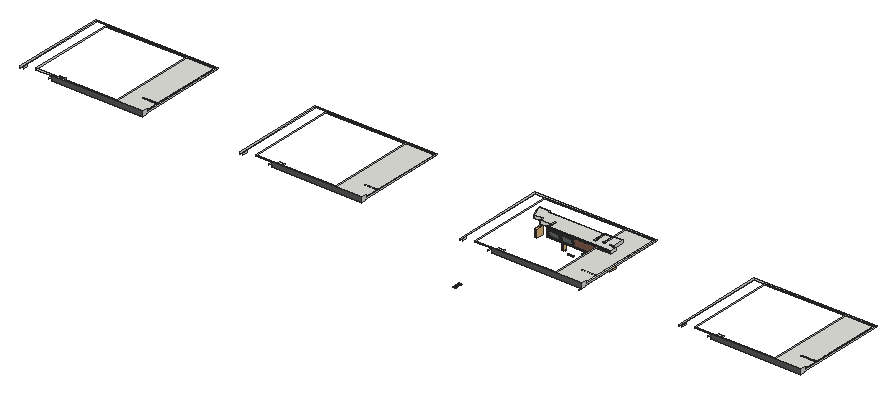
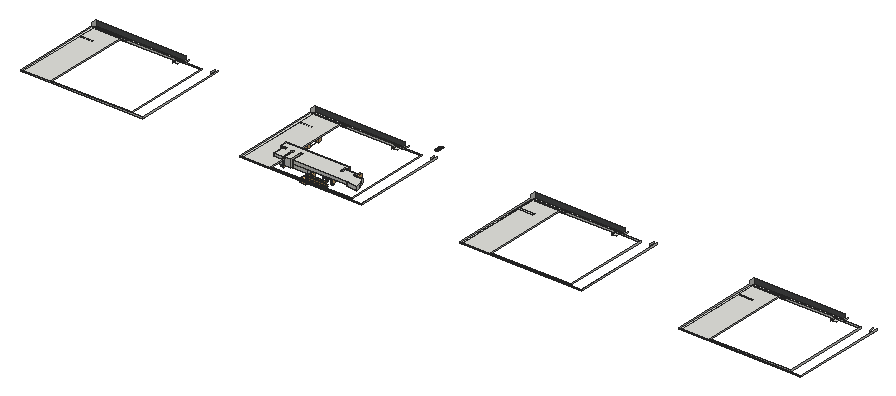
# SketchUp Ruby script. Lengths in inches.
U = 1.inch
M = Sketchup.active_model
def pt(a) = Geom::Point3d.new(a.map { |v| v * U })
def face(e, loops, mat)
  f = e.add_face(loops[0].map { |a| pt(a) })
  loops[1..].each { |l| e.add_face(l.map { |a| pt(a) }).erase! }
  f.material = f.back_material = mat if mat
  f
end
# faces: each face lists its corners as indices into pts; further lists are holes
def faces(e, pts, list, mat = nil) = list.each { |f| face(e, (f[0].is_a?(Array) ? f : [f]).map { |l| l.map { |i| pts[i] } }, mat) }
# xy, xz, yz: faces in a plane at the given z, y or x. An outline is a flat list of corners, or four numbers for a rectangle; further outlines are holes
def ring(l) = l.size == 4 ? [[l[0], l[1]], [l[2], l[1]], [l[2], l[3]], [l[0], l[3]]] : l.each_slice(2).to_a
def flat(e, list, mat, &to3) = list.each { |f| face(e, (f[0].is_a?(Array) ? f : [f]).map { |l| ring(l).map { |u, v| to3.(u, v) } }, mat) }
def xy(e, z, list, mat = nil) = flat(e, list, mat) { |x, y| [x, y, z] }
def xz(e, y, list, mat = nil) = flat(e, list, mat) { |x, z| [x, y, z] }
def yz(e, x, list, mat = nil) = flat(e, list, mat) { |y, z| [x, y, z] }
def lines(e, pts, list) = list.each { |a, b| e.add_line(pt(pts[a]), pt(pts[b])) }
# prism: a flat outline (further loops are holes) pulled along v
def prism(e, loops, v, mat = nil)
  f = face(e, loops, mat); d = Geom::Vector3d.new(v.map { |x| x * U })
  f.pushpull(f.normal.samedirection?(d) ? d.length : -d.length)
end
def box(e, o, s, mat = nil) = prism(e, [[o, [o[0] + s[0], o[1], o[2]], [o[0] + s[0], o[1] + s[1], o[2]], [o[0], o[1] + s[1], o[2]]]], [0, 0, s[2]], mat)
def at(x, y, z, deg = 0) = Geom::Transformation.translation(pt([x, y, z])) * Geom::Transformation.rotation(ORIGIN, Z_AXIS, deg.degrees)
def axes(o, x, y, z) = Geom::Transformation.new([*x, 0, *y, 0, *z, 0, *pt(o).to_a, 1])
def part(name) = M.definitions.add(name)
# library, detail: a bought-in or finely detailed component or shape, given as its bounding box
def library(name, o, s) = part(name).tap { |d| box(d.entities, o, s) }
def detail(e, o, s) = box(e.add_group.entities, o, s)
def put(e, d, t, mat = nil) = e.add_instance(d, t).tap { |i| i.material = mat if mat }
def group(e, t, mat = nil) = e.add_group.tap { |g| g.transformation = t; g.material = mat if mat }.entities
root = M.entities
M.materials.add("Aluminum_Polished").color = [83, 85, 85]
M.materials.add("Floor board").color = [119, 86, 70]
M.materials.add("Floor board2").color = [119, 86, 70]
M.materials.add("Image2").color = [96, 104, 104]
M.materials.add("Material31 copy1").color = [126, 98, 61]
M.materials.add("Small-Wooden-Floor").color = [116, 79, 55]
M.materials.add("Sophie_Shoes2").color = [35, 35, 35]
M.materials.add("[Metal_Corrogated_Shiny]2").color = [193, 193, 193]
M.materials.add("s500 white").color = [237, 237, 230]
c1 = library("IKEA FINTORP-",[6.23,0.25,8.28],[1.42,31.37,3.33])
c2 = library("ZJ8P4AC",[-1.97,-16.1,36],[20.97,16.1,19.66])
c3 = library("Group\#84",[0,-1.97,0],[16.33,39.37,11.37])
c4 = part("Component\#73")
detail(c4.entities,[0,0,-0.5],[5.95,16.95,0.625])
c5 = part("omponent_2\#3")
xy(c5.entities,0.125,[[[0.47,0.47,5.47,16.47],[1.375,15.02,4.5625,15.45],[1.375,14.15,4.5625,14.59],[1.375,13.29,4.5625,13.72],[1.375,12.43,4.5625,12.86],[1.375,11.5625,4.5625,12],[1.375,10.7,4.5625,11.13],[1.375,9.84,4.5625,10.27],[1.375,8.97,4.5625,9.41],[1.375,8.11,4.5625,8.54],[1.375,7.25,4.5625,7.68],[1.375,6.38,4.5625,6.82],[1.375,5.52,4.5625,5.95],[1.375,4.66,4.5625,5.09],[1.375,3.79,4.5625,4.23],[1.375,2.93,4.5625,3.36],[1.375,2.07,4.5625,2.5],[1.375,1.26,4.5625,1.64]]],"[Metal_Corrogated_Shiny]2")
put(c5.entities,c4,at(0,0,0))
c6 = library("Cobra Beer Dispense Font",[-3.83,-2.55,-1.15],[8.17,12.19,26.9])
c7 = library("maq caf expresso 2 mdulos",[-0.08,-0.31,0.08],[34.26,25.22,21.95])
c8 = library("Group\#83",[-2.91,0,0],[33.89,3.125,48.37])
c9 = part("Group\#60")
xy(c9.entities,0,[[-106.3,12.99,7.875,25.59]])
xy(c9.entities,1.97,[[-106.3,12.99,7.875,25.59]],"Material31 copy1")
xz(c9.entities,12.99,[[-106.3,0,7.875,1.97]],"Material31 copy1")
xz(c9.entities,25.59,[[-106.3,0,7.875,1.97]])
yz(c9.entities,-106.3,[[12.99,0,25.59,1.97]],"Material31 copy1")
yz(c9.entities,7.875,[[12.99,0,25.59,1.97]],"Material31 copy1")
c10 = library("Group\#105",[0,0,0],[37.34,15.24,44.88])
c11 = library("Group\#93",[0,0,0],[37.3,15.24,44.88])
c12 = library("Group\#94",[0,0,0],[37.3,15.24,44.88])
c13 = library("Group\#90",[0,0,0],[37.3,15.24,44.88])
c14 = part("Group\#62")
box(c14.entities,[0,-3.9375,0],[1.97,3.9375,1.97],"Sophie_Shoes2")
xy(root,120.25,[[492.21,559.875,492.21,581.125,527.2,581.125,527.2,589.17,810.34,589.17,810.34,581.125,1005.5,581.125,1005.5,559.875],[1742.84,559.875,1742.84,581.125,1777.83,581.125,1777.83,589.17,2060.96,589.17,2060.96,581.125,2256.12,581.125,2256.12,559.875],[2993.46,559.875,2993.46,581.125,3028.45,581.125,3028.45,589.17,3311.59,589.17,3311.59,581.125,3506.75,581.125,3506.75,559.875],[4244.09,559.875,4244.09,581.125,4279.08,581.125,4279.08,589.17,4562.21,589.17,4562.21,581.125,4757.37,581.125,4757.37,559.875],[810.34,581.125,939.09,589.17],
  [2060.96,581.125,2189.71,589.17],[3311.59,581.125,3440.34,589.17],[4562.21,581.125,4690.96,589.17]])
xy(root,126,[[310,559.875,313.69,1096.5],[1560.62,559.875,1564.31,1096.5],[2811.25,559.875,2814.94,1096.5],[4061.87,559.875,4065.56,1096.5],[810.34,581.125,990.19,589.17],
  [990.19,581.125,1005.5,589.17],[2060.96,581.125,2240.81,589.17],[2240.81,581.125,2256.12,589.17],[3311.59,581.125,3491.44,589.17],[3491.44,581.125,3506.75,589.17],
  [4562.21,581.125,4742.06,589.17],[4742.06,581.125,4757.37,589.17],[494.4,589.17,519.08,610.99],[519.08,589.17,527.2,610.99],[835.39,589.17,835.39,1088.45,989.64,1088.45,989.64,690.16,909.32,690.16,909.32,682.59,989.64,682.59,989.64,589.17],
  [989.64,589.17,989.64,682.59,909.32,682.59,909.32,690.16,989.64,690.16,989.64,1088.45,990.19,1088.45,990.19,589.17],[990.19,589.17,1005.5,1088.45],[1745.02,589.17,1769.7,610.99],[1769.7,589.17,1777.83,610.99],[2086.01,589.17,2086.01,1088.45,2240.26,1088.45,2240.26,690.16,2159.95,690.16,2159.95,682.59,2240.26,682.59,2240.26,589.17],
  [2240.26,589.17,2240.26,682.59,2159.95,682.59,2159.95,690.16,2240.26,690.16,2240.26,1088.45,2240.81,1088.45,2240.81,589.17],[2240.81,589.17,2256.12,1088.45],[2995.65,589.17,3020.33,610.99],[3020.33,589.17,3028.45,610.99],[3336.64,589.17,3336.64,1088.45,3490.89,1088.45,3490.89,690.16,3410.57,690.16,3410.57,682.59,3490.89,682.59,3490.89,589.17],
  [3490.89,589.17,3490.89,682.59,3410.57,682.59,3410.57,690.16,3490.89,690.16,3490.89,1088.45,3491.44,1088.45,3491.44,589.17],[3491.44,589.17,3506.75,1088.45],[4246.27,589.17,4270.95,610.99],[4270.95,589.17,4279.08,610.99],[4587.26,589.17,4587.26,1088.45,4741.51,1088.45,4741.51,690.16,4661.2,690.16,4661.2,682.59,4741.51,682.59,4741.51,589.17],
  [4741.51,589.17,4741.51,682.59,4661.2,682.59,4661.2,690.16,4741.51,690.16,4741.51,1088.45,4742.06,1088.45,4742.06,589.17],[4742.06,589.17,4757.37,1088.45],[990.19,1088.45,1005.5,1096.5],[2240.81,1088.45,2256.12,1096.5],[3491.44,1088.45,3506.75,1096.5],
  [4742.06,1088.45,4757.37,1096.5]])
xz(root,559.875,[[492.21,120.25,1005.5,148.4375],[1742.84,120.25,2256.12,148.4375],[2993.46,120.25,3506.75,148.4375],[4244.09,120.25,4757.37,148.4375]],"Aluminum_Polished")
xz(root,581.125,[[492.21,120.25,519.08,126],[810.34,120.25,990.19,126],[990.19,120.25,1005.5,126],[1742.84,120.25,1769.7,126],[2060.96,120.25,2240.81,126],
  [2240.81,120.25,2256.12,126],[2993.46,120.25,3020.33,126],[3311.59,120.25,3491.44,126],[3491.44,120.25,3506.75,126],[4244.09,120.25,4270.95,126],
  [4562.21,120.25,4742.06,126],[4742.06,120.25,4757.37,126]])
xz(root,589.17,[[527.2,120.25,527.2,126,376.61,126,376.61,132,835.39,132,835.39,126,810.34,126,810.34,120.25],[1777.83,120.25,1777.83,126,1627.23,126,1627.23,132,2086.01,132,2086.01,126,2060.96,126,2060.96,120.25],[3028.45,120.25,3028.45,126,2877.86,126,2877.86,132,3336.64,132,3336.64,126,3311.59,126,3311.59,120.25],[4279.08,120.25,4279.08,126,4128.48,126,4128.48,132,4587.26,132,4587.26,126,4562.21,126,4562.21,120.25]])
xz(root,1088.45,[[376.61,126,835.39,132],[1627.23,126,2086.01,132],[2877.86,126,3336.64,132],[4128.48,126,4587.26,132]])
xz(root,1096.5,[[310,126,1005.5,132],[1560.62,126,2256.12,132],[2811.25,126,3506.75,132],[4061.87,126,4757.37,132]])
yz(root,310,[[559.875,126,1096.5,132]])
yz(root,327.6,[[559.875,126,586.25,132]])
yz(root,376.61,[[589.17,126,1088.45,132]])
yz(root,474.41,[[559.875,126,586.25,132]])
yz(root,492.21,[[559.875,120.25,581.125,126]])
yz(root,527.2,[[589.17,120.25,610.99,126]])
yz(root,810.34,[[581.125,120.25,589.17,126]])
yz(root,835.39,[[589.17,126,1088.45,132]])
yz(root,1005.5,[[559.875,120.25,581.125,120.25,581.125,126,1096.5,126,1096.5,132,589.17,132,589.17,148.4375,559.875,148.4375]])
yz(root,1560.62,[[559.875,126,1096.5,132]])
yz(root,1578.23,[[559.875,126,586.25,132]])
yz(root,1627.23,[[589.17,126,1088.45,132]])
yz(root,1725.04,[[559.875,126,586.25,132]])
yz(root,1742.84,[[559.875,120.25,581.125,126]])
yz(root,1777.83,[[589.17,120.25,610.99,126]])
yz(root,2060.96,[[581.125,120.25,589.17,126]])
yz(root,2086.01,[[589.17,126,1088.45,132]])
yz(root,2256.12,[[559.875,120.25,581.125,120.25,581.125,126,1096.5,126,1096.5,132,589.17,132,589.17,148.4375,559.875,148.4375]])
yz(root,2811.25,[[559.875,126,1096.5,132]])
yz(root,2828.85,[[559.875,126,586.25,132]])
yz(root,2877.86,[[589.17,126,1088.45,132]])
yz(root,2975.66,[[559.875,126,586.25,132]])
yz(root,2993.46,[[559.875,120.25,581.125,126]])
yz(root,3028.45,[[589.17,120.25,610.99,126]])
yz(root,3311.59,[[581.125,120.25,589.17,126]])
yz(root,3336.64,[[589.17,126,1088.45,132]])
yz(root,3506.75,[[559.875,120.25,581.125,120.25,581.125,126,1096.5,126,1096.5,132,589.17,132,589.17,148.4375,559.875,148.4375]])
yz(root,4061.87,[[559.875,126,1096.5,132]])
yz(root,4079.48,[[559.875,126,586.25,132]])
yz(root,4128.48,[[589.17,126,1088.45,132]])
yz(root,4226.29,[[559.875,126,586.25,132]])
yz(root,4244.09,[[559.875,120.25,581.125,126]])
yz(root,4279.08,[[589.17,120.25,610.99,126]])
yz(root,4562.21,[[581.125,120.25,589.17,126]])
yz(root,4587.26,[[589.17,126,1088.45,132]])
yz(root,4757.37,[[559.875,120.25,581.125,120.25,581.125,126,1096.5,126,1096.5,132,589.17,132,589.17,148.4375,559.875,148.4375]])
p = [[3020.33,581.125,126],[3020.33,589.17,126],[3214.14,581.125,126],[3308.27,581.125,126],[3311.2,581.125,126],[4558.89,581.125,126],
  [4561.83,581.125,126],[4464.77,581.125,126],[4270.95,581.125,126],[4270.95,589.17,126],[807.02,581.125,126],[809.95,581.125,126],
  [712.89,581.125,126],[519.08,581.125,126],[519.08,589.17,126],[1769.7,581.125,126],[1963.52,581.125,126],[1769.7,589.17,126],
  [2057.64,581.125,126],[2060.58,581.125,126],[3414.37,657.41,85.63],[3414.37,657.41,86.42]]
lines(root,p,[[0,1],[0,2],[2,3],[3,4],[5,6],[7,5],[8,7],[8,9],[10,11],[12,10],[13,12],[13,14],
  [15,16],[15,17],[18,19],[16,18],[20,21]])
put(root,c1,at(3202.59,879.08,23.11,90))
put(root,c2,at(3254.94,899.29,-4.5,180))
put(root,c3,at(3398.04,881.87,31.5))
g1 = group(root,at(2970.57,380.49,32.37,-179.359))
p = [[0.32,2.1875,0.18],[7.39,3.76,0.59],[-0.4,2.38,0.15],[-0.93,2.91,0.125],[-1.12,3.625,0.16],[-0.93,41.52,0.125],
  [-1.12,40.8,0.16],[7.39,40.67,0.59],[-0.4,42.05,0.15],[0.32,42.24,0.18],[7.63,2.1875,0.45],[6.64,10.92,0.99],
  [-1.12,10.92,0.7],[-1.12,33.51,0.7],[6.64,33.51,0.99],[7.63,42.24,0.45],[16.47,2.1875,0.53],[16.47,42.24,0.53],
  [17.1875,2.38,0.55],[17.72,2.91,0.59],[17.1875,42.05,0.55],[17.72,41.52,0.59],[17.91,3.63,0.63],[17.91,10.92,1.1],
  [17.91,40.8,0.63],[17.91,33.51,1.1],[6.17,22.21,1.12],[-1.12,22.21,0.92],[17.91,22.21,1.22]]
faces(g1,p,[[0,1,2],[3,2,1],[4,3,1],[5,6,7],[8,5,7],[7,9,8],[1,0,10],[1,11,4],
  [12,4,11],[6,13,14],[14,7,6],[9,7,15],[10,16,1],[17,15,7],[1,19,22],[11,22,23],
  [11,1,22],[7,14,24],[24,14,25],[21,7,24],[26,27,12],[26,12,11],[27,26,13],[13,26,14],
  [26,11,23],[14,26,25],[26,23,28],[25,26,28]],"s500 white")
faces(g1,p,[[18,1,16],[1,18,19],[20,7,21],[7,20,17]])
put(root,c5,at(3122.85,910,35.43,-90))
put(root,c6,at(3131.53,899.51,36.59))
put(root,c7,at(3217.125,963.11,37.4))
g2 = group(root,at(3414.37,696.25,39.37))
prism(g2,[[[0,-38.84,0.2],[0,-38.84,0],[0.79,-38.84,0],[0.79,-38.84,1.18],[0,-38.84,1.18],[0,-38.84,0.98],[0.59,-38.84,0.98],[0.59,-38.84,0.2]]],[0,261.86,0],"Sophie_Shoes2")
put(root,c8,axes([3415.04,889.76,52.09],[0,0.73,0],[-0.73,0,0],[0,0,0.73]))
put(root,c9,at(3207.1875,963.11,59.84))
put(root,c10,at(3377.21,681.92,68.23))
put(root,c11,at(3377.21,756.72,68.23))
put(root,c12,at(3377.21,831.52,68.23))
put(root,c13,at(3010.52,864.78,68.9,90))
put(root,c9,at(3207.1875,963.11,72.24))
g3 = group(root,at(3414.37,657.41,85.43))
prism(g3,[[[0,0,0.2],[0,0,0],[0.79,0,0],[0.79,0,1.18],[0,0,1.18],[0,0,0.98],[0.59,0,0.98],[0.59,0,0.2]]],[0,261.86,0],"Sophie_Shoes2")
g4 = group(root,at(3062.21,902.08,137.8))
xy(g4,-52.36,[[[-9.84,-21.65,-9.84,0,0,0,0,-11.8125,352.95,-11.8125,352.95,-21.65],[0,-20.47,195.18,-12.99]]],"Sophie_Shoes2")
xy(g4,-51.38,[[-9.84,-21.65,-9.25,0],[-9.25,-21.65,352.95,-21.0625]],"Sophie_Shoes2")
xy(g4,-51.18,[[-9.84,-21.65,-9.84,0,-9.25,0,-9.25,-21.0625,352.95,-21.0625,352.95,-21.65]],"Floor board")
xy(g4,-51.18,[[0,-12.4,145.18,-11.8125]],"Sophie_Shoes2")
xy(g4,-50.59,[[0,-12.4,145.18,-11.8125]])
xy(g4,-47.64,[[0,-20.47,195.18,-12.99]],"Sophie_Shoes2")
xy(g4,-43.31,[[145.18,-11.8125,145.18,86.61,231.79,86.61,231.79,13.78,242,13.78,242,27.56,237.7,27.56,237.7,86.61,277.8,86.61,277.8,27.56,273.49,27.56,273.49,21.65,285.85,21.65,285.85,27.56,283.7,27.56,283.7,92.52,335.25,92.52,335.25,27.56,317.35,27.56,317.35,21.65,330.23,21.65,330.23,17.19,352.95,17.19,352.95,-11.8125]])
xy(g4,-19.69,[[0,-11.8125,0,29.53,-5.91,29.53,-5.91,5.91,-68.9,5.91,-68.9,27.62,-120.71,27.62,-132.65,55.86,-137.96,70.69,-145.4,96.46,-84.48,96.46,-84.48,86.61,145.18,86.61,145.18,-11.8125]])
xy(g4,-6.3,[[-9.84,-21.65,352.95,-20.87],[-9.84,-20.87,-9.06,0]],"Small-Wooden-Floor")
xy(g4,0,[[-9.06,-20.87,352.95,-20.87,352.95,17.19,330.23,17.19,330.23,21.65,317.35,21.65,317.35,27.56,335.25,27.56,335.25,92.52,283.7,92.52,283.7,27.56,285.85,27.56,285.85,21.65,273.49,21.65,273.49,27.56,277.8,27.56,277.8,86.61,237.7,86.61,237.7,27.56,242,27.56,242,13.78,231.79,13.78,231.79,86.61,-84.48,86.61,-84.48,96.46,-145.4,96.46,-137.96,70.69,-132.65,55.86,-120.71,27.62,-68.9,27.62,-68.9,5.91,-5.91,5.91,-5.91,29.53,0,29.53,0,0,-9.06,0]])
xz(g4,-21.65,[[-9.84,-51.18,352.95,-6.3]],"Floor board")
xz(g4,-21.65,[[-9.84,-52.36,352.95,-51.38]],"Sophie_Shoes2")
xz(g4,-21.0625,[[-9.25,-51.38,352.95,-51.18]],"Sophie_Shoes2")
xz(g4,-20.87,[[-9.06,-6.3,352.95,0]],"Sophie_Shoes2")
xz(g4,-20.47,[[0,-52.36,195.18,-47.64]])
xz(g4,-12.99,[[0,-52.36,195.18,-47.64]],"Sophie_Shoes2")
xz(g4,-12.4,[[0,-51.18,145.18,-50.59]],"Sophie_Shoes2")
xz(g4,-11.8125,[[0,-50.59,145.18,-19.69]])
xz(g4,-11.8125,[[0,-52.36,0,-51.18,145.18,-51.18,145.18,-43.31,352.95,-43.31,352.95,-52.36]],"Sophie_Shoes2")
xz(g4,0,[[-9.84,-52.36,-9.84,-51.38,-9.25,-51.38,-9.25,-51.18,-9.84,-51.18,-9.84,-6.3,-9.06,-6.3,-9.06,0,0,0,0,-52.36]])
xz(g4,5.91,[[-68.9,-19.69,-5.91,0]])
xz(g4,13.78,[[231.79,-43.31,242,0]])
xz(g4,17.19,[[330.23,-43.31,352.95,0]])
xz(g4,21.65,[[273.49,-43.31,285.85,0],[317.35,-43.31,330.23,0]])
xz(g4,27.56,[[237.7,-43.31,242,0],[273.49,-43.31,277.8,0],[283.7,-43.31,285.85,0],[317.35,-43.31,335.25,0]])
xz(g4,27.62,[[-120.71,-19.69,-68.9,0]])
xz(g4,29.53,[[-5.91,-19.69,0,0]])
xz(g4,86.61,[[145.18,-43.31,231.79,-19.69],[237.7,-43.31,277.8,0],[-84.48,-19.69,231.79,0]])
xz(g4,92.52,[[283.7,-43.31,335.25,0]])
xz(g4,96.46,[[-145.4,-19.69,-84.48,0]])
yz(g4,-84.48,[[86.61,-19.69,96.46,0]])
yz(g4,-68.9,[[5.91,-19.69,27.62,0]])
yz(g4,-9.84,[[-21.65,-51.18,0,-6.3]],"Floor board2")
yz(g4,-9.84,[[-21.65,-52.36,0,-51.38]],"Sophie_Shoes2")
yz(g4,-9.25,[[-21.0625,-51.38,0,-51.18]],"Sophie_Shoes2")
yz(g4,-9.06,[[-20.87,-6.3,0,0]],"Sophie_Shoes2")
yz(g4,-5.91,[[5.91,-19.69,29.53,0]])
yz(g4,0,[[-11.8125,-52.36,0,-52.36,0,-19.69,-11.8125,-19.69,-11.8125,-50.59,-12.4,-50.59,-12.4,-51.18,-11.8125,-51.18],[0,-19.69,29.53,0]])
yz(g4,0,[[-20.47,-52.36,-12.99,-47.64]],"Sophie_Shoes2")
yz(g4,145.18,[[-12.4,-51.18,-11.8125,-50.59],[-11.8125,-43.31,86.61,-19.69]])
yz(g4,195.18,[[-20.47,-52.36,-12.99,-47.64]],"Sophie_Shoes2")
yz(g4,231.79,[[13.78,-43.31,86.61,-19.69],[13.78,-19.69,86.61,0]])
yz(g4,237.7,[[27.56,-43.31,86.61,0]])
yz(g4,242,[[13.78,-43.31,27.56,0]])
yz(g4,273.49,[[21.65,-43.31,27.56,0]])
yz(g4,277.8,[[27.56,-43.31,86.61,0]])
yz(g4,283.7,[[27.56,-43.31,92.52,0]])
yz(g4,285.85,[[21.65,-43.31,27.56,0]])
yz(g4,317.35,[[21.65,-43.31,27.56,0]])
yz(g4,330.23,[[17.19,-43.31,21.65,0]])
yz(g4,335.25,[[27.56,-43.31,92.52,0]])
yz(g4,352.95,[[-21.65,-52.36,-11.8125,-52.36,-11.8125,-43.31,17.19,-43.31,17.19,0,-20.87,0,-20.87,-6.3,-21.65,-6.3,-21.65,-51.18,-21.0625,-51.18,-21.0625,-51.38,-21.65,-51.38]])
p = [[-120.71,27.62,0],[-132.65,55.86,0],[-132.65,55.86,-19.69],[-120.71,27.62,-19.69],[-137.96,70.69,0],[-137.96,70.69,-19.69],
  [-145.4,96.46,0],[-145.4,96.46,-19.69],[352.95,-21.65,-6.3],[362.91,-21.65,-6.3]]
faces(g4,p,[[0,1,2,3],[1,4,5,2],[4,6,7,5]])
lines(g4,p,[[8,9]])
put(root,c9,at(3207.1875,963.11,85.43))
g5 = group(root,at(3136.83,875.16,89.68))
put(g5,c14,at(0,5.9,37.38))
g6 = group(g5,at(0,5.94,0.2))
yz(g6,0,[[-1.96,-0.2,-5.94,38.95,-3.98,39.15,0,0]],"Sophie_Shoes2")
yz(g6,1.97,[[-2.16,1.76,-1.96,1.78,-5.54,37.01,-5.74,36.99]],"Sophie_Shoes2")
yz(g6,64.96,[[-2.16,1.76,-5.74,36.99,-5.54,37.01,-1.96,1.78]],"Sophie_Shoes2")
yz(g6,66.93,[[-1.96,-0.2,0,0,-3.98,39.15,-5.94,38.95]],"Sophie_Shoes2")
p = [[0,-1.96,-0.2],[66.93,-1.96,-0.2],[66.93,-5.94,38.95],[0,-5.94,38.95],[64.96,-5.74,36.99],[64.96,-2.16,1.76],
  [1.97,-2.16,1.76],[1.97,-5.74,36.99],[0,0,0],[66.93,0,0],[0,-3.98,39.15],[66.93,-3.98,39.15],
  [64.96,-1.96,1.78],[64.96,-5.54,37.01],[1.97,-5.54,37.01],[1.97,-1.96,1.78]]
faces(g6,p,[[[0,1,2,3],[4,5,6,7]],[8,9,1,0],[9,8,10,11],[6,5,12,15],[4,7,14,13],[11,10,3,2]],"Sophie_Shoes2")
faces(g6,p,[[12,13,14,15]],"Image2")
put(g5,c14,at(64.96,5.9,37.38))
g7 = group(root,at(3062.1875,875.16,89.68))
put(g7,c14,at(0,5.9,37.38))
g8 = group(g7,at(0,5.94,0.2))
yz(g8,0,[[-1.96,-0.2,-5.94,38.95,-3.98,39.15,0,0]],"Sophie_Shoes2")
yz(g8,1.97,[[-2.16,1.76,-1.96,1.78,-5.54,37.01,-5.74,36.99]],"Sophie_Shoes2")
yz(g8,64.96,[[-2.16,1.76,-5.74,36.99,-5.54,37.01,-1.96,1.78]],"Sophie_Shoes2")
yz(g8,66.93,[[-1.96,-0.2,0,0,-3.98,39.15,-5.94,38.95]],"Sophie_Shoes2")
p = [[0,-1.96,-0.2],[66.93,-1.96,-0.2],[66.93,-5.94,38.95],[0,-5.94,38.95],[64.96,-5.74,36.99],[64.96,-2.16,1.76],
  [1.97,-2.16,1.76],[1.97,-5.74,36.99],[0,0,0],[66.93,0,0],[0,-3.98,39.15],[66.93,-3.98,39.15],
  [64.96,-1.96,1.78],[64.96,-5.54,37.01],[1.97,-5.54,37.01],[1.97,-1.96,1.78]]
faces(g8,p,[[[0,1,2,3],[4,5,6,7]],[8,9,1,0],[9,8,10,11],[6,5,12,15],[4,7,14,13],[11,10,3,2]],"Sophie_Shoes2")
faces(g8,p,[[12,13,14,15]],"Image2")
put(g7,c14,at(64.96,5.9,37.38))
